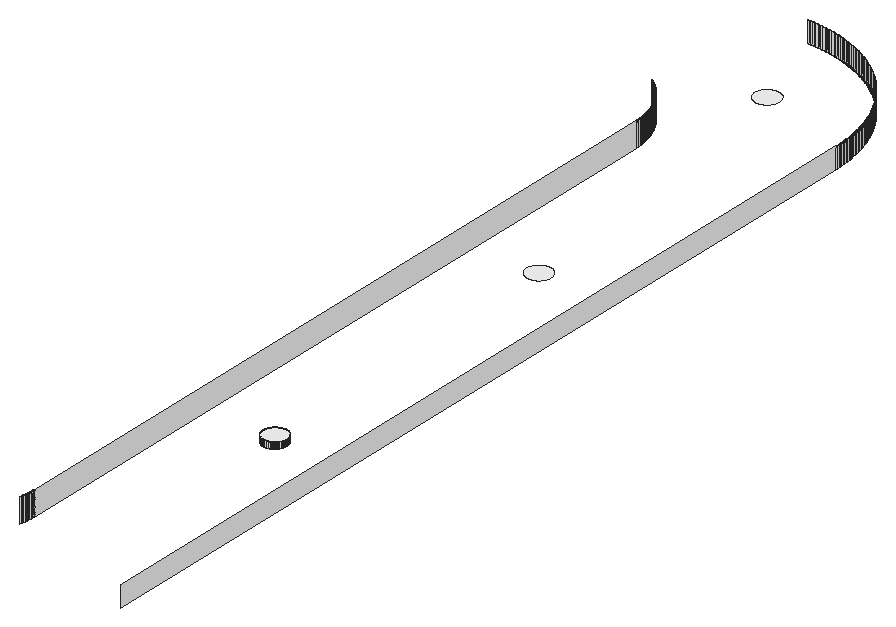
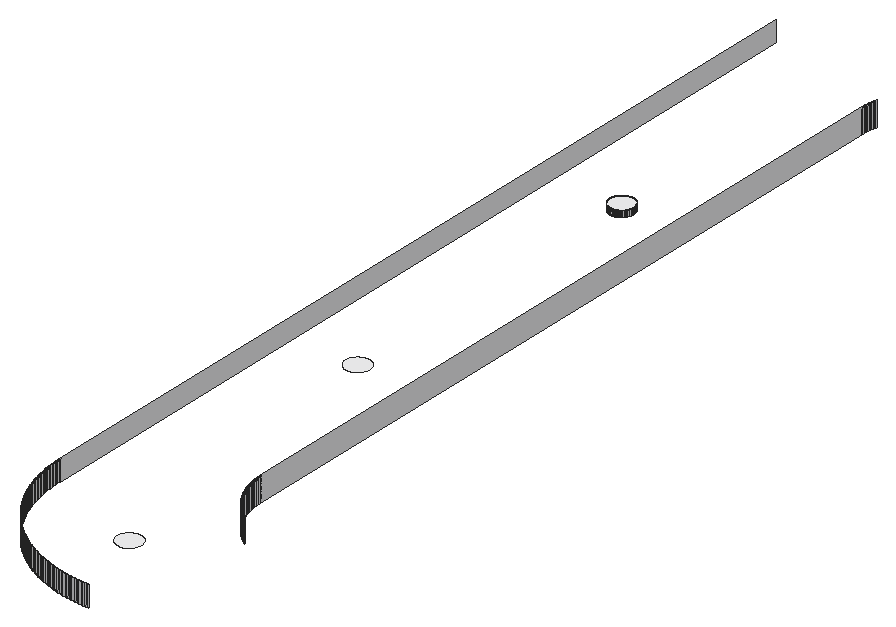
# SketchUp Ruby script. Lengths in inches.
U = 1.inch
M = Sketchup.active_model
def pt(a) = Geom::Point3d.new(a.map { |v| v * U })
def face(e, loops, mat)
  f = e.add_face(loops[0].map { |a| pt(a) })
  loops[1..].each { |l| e.add_face(l.map { |a| pt(a) }).erase! }
  f.material = f.back_material = mat if mat
  f
end
# faces: each face lists its corners as indices into pts; further lists are holes
def faces(e, pts, list, mat = nil) = list.each { |f| face(e, (f[0].is_a?(Array) ? f : [f]).map { |l| l.map { |i| pts[i] } }, mat) }
# xy, xz, yz: faces in a plane at the given z, y or x. An outline is a flat list of corners, or four numbers for a rectangle; further outlines are holes
def ring(l) = l.size == 4 ? [[l[0], l[1]], [l[2], l[1]], [l[2], l[3]], [l[0], l[3]]] : l.each_slice(2).to_a
def flat(e, list, mat, &to3) = list.each { |f| face(e, (f[0].is_a?(Array) ? f : [f]).map { |l| ring(l).map { |u, v| to3.(u, v) } }, mat) }
def xy(e, z, list, mat = nil) = flat(e, list, mat) { |x, y| [x, y, z] }
def xz(e, y, list, mat = nil) = flat(e, list, mat) { |x, z| [x, y, z] }
def yz(e, x, list, mat = nil) = flat(e, list, mat) { |y, z| [x, y, z] }
def lines(e, pts, list) = list.each { |a, b| e.add_line(pt(pts[a]), pt(pts[b])) }
# prism: a flat outline (further loops are holes) pulled along v
def prism(e, loops, v, mat = nil)
  f = face(e, loops, mat); d = Geom::Vector3d.new(v.map { |x| x * U })
  f.pushpull(f.normal.samedirection?(d) ? d.length : -d.length)
end
def box(e, o, s, mat = nil) = prism(e, [[o, [o[0] + s[0], o[1], o[2]], [o[0] + s[0], o[1] + s[1], o[2]], [o[0], o[1] + s[1], o[2]]]], [0, 0, s[2]], mat)
def at(x, y, z, deg = 0) = Geom::Transformation.translation(pt([x, y, z])) * Geom::Transformation.rotation(ORIGIN, Z_AXIS, deg.degrees)
def axes(o, x, y, z) = Geom::Transformation.new([*x, 0, *y, 0, *z, 0, *pt(o).to_a, 1])
def part(name) = M.definitions.add(name)
# library, detail: a bought-in or finely detailed component or shape, given as its bounding box
def library(name, o, s) = part(name).tap { |d| box(d.entities, o, s) }
def detail(e, o, s) = box(e.add_group.entities, o, s)
def put(e, d, t, mat = nil) = e.add_instance(d, t).tap { |i| i.material = mat if mat }
def group(e, t, mat = nil) = e.add_group.tap { |g| g.transformation = t; g.material = mat if mat }.entities
root = M.entities
M.materials.add("[Quartz Light Grey]").color = [251, 251, 252]
xy(root,112.81,[[188.98,111.35,188.85,111.36,188.73,111.37,188.6,111.39,188.48,111.42,188.24,111.5,188.13,111.55,188.02,111.61,187.91,111.68,187.81,111.75,187.71,111.83,187.62,111.91,187.53,112,187.37,112.2,187.3,112.3,187.18,112.52,187.13,112.64,187.09,112.76,187.03,113,187.01,113.125,187,113.25,187,113.375,187.02,113.625,187.04,113.75,187.1,113.99,187.2,114.23,187.26,114.34,187.32,114.44,187.39,114.55,187.47,114.65,187.65,114.83,187.74,114.91,187.84,114.98,188.06,115.12,188.28,115.22,188.52,115.3,188.65,115.32,188.77,115.34,188.9,115.35,189.15,115.35,189.27,115.34,189.4,115.31,189.52,115.29,189.76,115.21,189.87,115.15,189.98,115.1,190.09,115.03,190.19,114.96,190.29,114.88,190.38,114.8,190.47,114.71,190.63,114.51,190.7,114.41,190.76,114.3,190.82,114.1875,190.87,114.07,190.91,113.95,190.97,113.71,190.99,113.58,191,113.46,191,113.33,190.99,113.21,190.98,113.08,190.96,112.96,190.9,112.72,190.8,112.48,190.68,112.26,190.61,112.16,190.53,112.0625,190.44,111.97,190.35,111.88,190.26,111.8,190.16,111.72,190.05,111.65,189.94,111.59,189.72,111.49,189.48,111.41,189.35,111.39,189.23,111.37,189.1,111.36],[188.85,166.71,188.73,166.73,188.6,166.75,188.48,166.78,188.36,166.8125,188.24,166.86,188.13,166.91,187.91,167.03,187.81,167.1,187.71,167.18,187.53,167.36,187.45,167.45,187.37,167.55,187.3,167.66,187.24,167.76,187.18,167.875,187.13,167.99,187.09,168.11,187.03,168.35,187.01,168.48,187,168.6,187,168.73,187.01,168.86,187.02,168.98,187.04,169.1,187.07,169.23,187.1,169.35,187.15,169.46,187.2,169.58,187.32,169.8,187.39,169.9,187.47,170,187.65,170.18,187.74,170.26,187.84,170.34,187.95,170.41,188.17,170.53,188.28,170.58,188.4,170.62,188.52,170.65,188.65,170.68,188.77,170.7,188.9,170.71,189.02,170.71,189.15,170.7,189.27,170.69,189.4,170.67,189.52,170.64,189.76,170.56,189.87,170.51,190.09,170.39,190.19,170.3125,190.29,170.24,190.38,170.15,190.47,170.0625,190.55,169.97,190.63,169.87,190.7,169.76,190.82,169.54,190.87,169.42,190.91,169.31,190.94,169.19,190.97,169.0625,190.99,168.9375,191,168.8125,191,168.6875,190.98,168.4375,190.96,168.3125,190.93,168.19,190.9,168.07,190.85,167.95,190.8,167.84,190.68,167.62,190.61,167.52,190.53,167.42,190.44,167.32,190.35,167.24,190.26,167.15,190.16,167.08,190.05,167.01,189.83,166.89,189.72,166.84,189.6,166.8,189.48,166.77,189.35,166.74,189.23,166.72,189.1,166.71],[182.98,222.0625,182.85,222.07,182.73,222.08,182.6,222.1,182.48,222.13,182.24,222.21,182.13,222.26,182.02,222.32,181.91,222.39,181.81,222.46,181.71,222.54,181.62,222.62,181.53,222.71,181.45,222.8,181.37,222.9,181.3,223.01,181.18,223.23,181.13,223.35,181.09,223.47,181.03,223.71,181.01,223.83,181,223.96,181,224.08,181.01,224.21,181.02,224.33,181.04,224.46,181.1,224.7,181.15,224.82,181.2,224.93,181.26,225.05,181.32,225.15,181.39,225.26,181.47,225.35,181.56,225.45,181.65,225.54,181.74,225.62,181.84,225.69,182.06,225.83,182.28,225.93,182.52,226.01,182.65,226.03,182.77,226.05,182.9,226.06,183.02,226.0625,183.15,226.06,183.27,226.04,183.4,226.02,183.64,225.96,183.76,225.91,183.87,225.86,184.09,225.74,184.19,225.67,184.29,225.59,184.38,225.51,184.47,225.42,184.63,225.22,184.7,225.12,184.76,225.01,184.82,224.89,184.87,224.78,184.91,224.66,184.97,224.42,184.99,224.29,185,224.17,185,224.04,184.99,223.92,184.98,223.79,184.96,223.67,184.93,223.54,184.9,223.42,184.85,223.31,184.8,223.19,184.68,222.97,184.61,222.87,184.53,222.77,184.35,222.59,184.26,222.51,184.16,222.43,184.05,222.36,183.83,222.24,183.72,222.2,183.6,222.15,183.48,222.12,183.35,222.09,183.23,222.08,183.1,222.07]],"[Quartz Light Grey]")
xz(root,115.35,[[188.9,111.81,189.02,112.81],[189.02,111.81,189.15,112.81]],"[Quartz Light Grey]")
xz(root,239.99,[[177.5,111.81,177.75,115.32]],"[Quartz Light Grey]")
xz(root,240,[[177,111.81,177.25,115.32]],"[Quartz Light Grey]")
yz(root,177,[[77.6875,111.81,77.84,115.91],[77.84,111.81,78,115.91],[78,111.81,204,115.91],[204,111.81,204.16,115.91],[204.16,111.81,204.3125,115.91]],"[Quartz Light Grey]")
yz(root,187,[[113.25,111.81,113.375,112.81]],"[Quartz Light Grey]")
yz(root,191,[[113.33,111.81,113.46,112.81]],"[Quartz Light Grey]")
yz(root,200.99,[[216.5,111.81,216.75,115.32]],"[Quartz Light Grey]")
yz(root,201,[[66,111.81,216,115.32],[216,111.81,216.25,115.32]],"[Quartz Light Grey]")
p = [[176.74,75.51,111.81],[176.7,75.35,111.81],[176.7,75.35,115.91],[176.74,75.51,115.91],[176.77,75.66,111.81],[176.77,75.66,115.91],
  [176.8,75.8125,111.81],[176.8,75.8125,115.91],[176.83,75.97,111.81],[176.83,75.97,115.91],[176.85,76.12,111.81],[176.85,76.12,115.91],
  [176.875,76.28,111.81],[176.875,76.28,115.91],[176.9,76.43,111.81],[176.9,76.43,115.91],[176.92,76.59,111.81],[176.92,76.59,115.91],
  [176.93,76.75,111.81],[176.93,76.75,115.91],[176.95,76.9,111.81],[176.95,76.9,115.91],[176.96,77.06,111.81],[176.96,77.06,115.91],
  [176.97,77.22,111.81],[176.97,77.22,115.91],[176.98,77.37,111.81],[176.98,77.37,115.91],[176.99,77.53,111.81],[176.99,77.53,115.91],
  [177,77.6875,111.81],[177,77.6875,115.91],[188.48,111.42,111.81],[188.36,111.46,111.81],[188.36,111.46,112.81],[188.48,111.42,112.81],
  [188.6,111.39,111.81],[188.6,111.39,112.81],[188.73,111.37,111.81],[188.73,111.37,112.81],[188.85,111.36,111.81],[188.85,111.36,112.81],
  [188.98,111.35,111.81],[188.98,111.35,112.81],[189.1,111.36,111.81],[189.1,111.36,112.81],[189.23,111.37,111.81],[189.23,111.37,112.81],
  [189.35,111.39,111.81],[189.35,111.39,112.81],[189.48,111.41,111.81],[189.48,111.41,112.81],[189.6,111.45,111.81],[189.6,111.45,112.81],
  [189.72,111.49,111.81],[189.72,111.49,112.81],[188.24,111.5,111.81],[188.13,111.55,111.81],[188.13,111.55,112.81],[188.24,111.5,112.81],
  [189.83,111.54,111.81],[189.83,111.54,112.81],[189.94,111.59,111.81],[189.94,111.59,112.81],[188.02,111.61,111.81],[187.91,111.68,111.81],
  [187.91,111.68,112.81],[188.02,111.61,112.81],[190.05,111.65,111.81],[190.05,111.65,112.81],[187.81,111.75,111.81],[187.71,111.83,111.81],
  [187.71,111.83,112.81],[187.81,111.75,112.81],[190.16,111.72,111.81],[190.16,111.72,112.81],[190.26,111.8,111.81],[190.26,111.8,112.81],
  [187.62,111.91,111.81],[187.62,111.91,112.81],[190.35,111.88,111.81],[190.35,111.88,112.81],[187.53,112,111.81],[187.53,112,112.81],
  [190.44,111.97,111.81],[190.44,111.97,112.81],[187.45,112.1,111.81],[187.45,112.1,112.81],[190.53,112.0625,111.81],[190.53,112.0625,112.81],
  [187.37,112.2,111.81],[187.37,112.2,112.81],[190.61,112.16,111.81],[190.61,112.16,112.81],[187.3,112.3,111.81],[187.3,112.3,112.81],
  [190.68,112.26,111.81],[190.68,112.26,112.81],[187.24,112.41,111.81],[187.24,112.41,112.81],[190.74,112.37,111.81],[190.74,112.37,112.81],
  [187.18,112.52,111.81],[187.18,112.52,112.81],[190.8,112.48,111.81],[190.8,112.48,112.81],[187.13,112.64,111.81],[187.13,112.64,112.81],
  [190.85,112.6,111.81],[190.85,112.6,112.81],[187.09,112.76,111.81],[187.09,112.76,112.81],[190.9,112.72,111.81],[190.9,112.72,112.81],
  [190.93,112.84,111.81],[190.93,112.84,112.81],[187.06,112.88,111.81],[187.06,112.88,112.81],[190.96,112.96,111.81],[190.96,112.96,112.81],
  [187.03,113,111.81],[187.03,113,112.81],[187.01,113.125,111.81],[187.01,113.125,112.81],[190.98,113.08,111.81],[190.98,113.08,112.81],
  [187,113.25,111.81],[187,113.25,112.81],[190.99,113.21,111.81],[190.99,113.21,112.81],[191,113.33,111.81],[191,113.33,112.81],
  [187,113.375,111.81],[187.01,113.5,111.81],[187.01,113.5,112.81],[187,113.375,112.81],[187.02,113.625,111.81],[187.02,113.625,112.81],
  [190.99,113.58,111.81],[191,113.46,111.81],[191,113.46,112.81],[190.99,113.58,112.81],[187.04,113.75,111.81],[187.04,113.75,112.81],
  [190.97,113.71,111.81],[190.97,113.71,112.81],[190.94,113.83,111.81],[190.94,113.83,112.81],[187.07,113.87,111.81],[187.07,113.87,112.81],
  [190.91,113.95,111.81],[190.91,113.95,112.81],[187.1,113.99,111.81],[187.1,113.99,112.81],[187.15,114.11,111.81],[187.15,114.11,112.81],
  [190.87,114.07,111.81],[190.87,114.07,112.81],[187.2,114.23,111.81],[187.2,114.23,112.81],[190.82,114.1875,111.81],[190.82,114.1875,112.81],
  [187.26,114.34,111.81],[187.26,114.34,112.81],[190.76,114.3,111.81],[190.76,114.3,112.81],[187.32,114.44,111.81],[187.32,114.44,112.81],
  [190.7,114.41,111.81],[190.7,114.41,112.81],[187.39,114.55,111.81],[187.39,114.55,112.81],[190.63,114.51,111.81],[190.63,114.51,112.81],
  [187.47,114.65,111.81],[187.47,114.65,112.81],[190.55,114.61,111.81],[190.55,114.61,112.81],[187.56,114.74,111.81],[187.56,114.74,112.81],
  [190.47,114.71,111.81],[190.47,114.71,112.81],[187.65,114.83,111.81],[187.65,114.83,112.81],[190.38,114.8,111.81],[190.38,114.8,112.81],
  [187.74,114.91,111.81],[187.74,114.91,112.81],[190.29,114.88,111.81],[190.29,114.88,112.81],[187.84,114.98,111.81],[187.84,114.98,112.81],
  [190.19,114.96,111.81],[190.19,114.96,112.81],[187.95,115.05,111.81],[187.95,115.05,112.81],[189.98,115.1,111.81],[190.09,115.03,111.81],
  [190.09,115.03,112.81],[189.98,115.1,112.81],[188.06,115.12,111.81],[188.06,115.12,112.81],[188.17,115.17,111.81],[188.17,115.17,112.81],
  [189.87,115.15,111.81],[189.87,115.15,112.81],[188.28,115.22,111.81],[188.28,115.22,112.81],[188.4,115.26,111.81],[188.4,115.26,112.81],
  [189.52,115.29,111.81],[189.64,115.25,111.81],[189.64,115.25,112.81],[189.52,115.29,112.81],[189.76,115.21,111.81],[189.76,115.21,112.81],
  [188.52,115.3,111.81],[188.52,115.3,112.81],[188.65,115.32,111.81],[188.65,115.32,112.81],[188.77,115.34,111.81],[188.77,115.34,112.81],
  [188.9,115.35,111.81],[188.9,115.35,112.81],[189.15,115.35,111.81],[189.27,115.34,111.81],[189.27,115.34,112.81],[189.15,115.35,112.81],
  [189.4,115.31,111.81],[189.4,115.31,112.81],[176.99,204.47,111.81],[177,204.3125,111.81],[177,204.3125,115.91],[176.99,204.47,115.91],
  [176.98,204.63,111.81],[176.98,204.63,115.91],[176.97,204.78,111.81],[176.97,204.78,115.91],[176.96,204.94,111.81],[176.96,204.94,115.91],
  [176.95,205.1,111.81],[176.95,205.1,115.91],[176.93,205.25,111.81],[176.93,205.25,115.91],[176.92,205.41,111.81],[176.92,205.41,115.91],
  [176.9,205.57,111.81],[176.9,205.57,115.91],[176.875,205.72,111.81],[176.875,205.72,115.91],[176.85,205.88,111.81],[176.85,205.88,115.91],
  [176.83,206.03,111.81],[176.83,206.03,115.91],[176.8,206.1875,111.81],[176.8,206.1875,115.91],[176.77,206.34,111.81],[176.77,206.34,115.91],
  [176.74,206.49,111.81],[176.74,206.49,115.91],[176.7,206.65,111.81],[176.7,206.65,115.91],[176.67,206.8,111.81],[176.67,206.8,115.91],
  [176.63,206.95,111.81],[176.63,206.95,115.91],[176.59,207.11,111.81],[176.59,207.11,115.91],[176.55,207.26,111.81],[176.55,207.26,115.91],
  [176.51,207.41,111.81],[176.51,207.41,115.91],[176.46,207.56,111.81],[176.46,207.56,115.91],[176.41,207.71,111.81],[176.41,207.71,115.91],
  [176.36,207.86,111.81],[176.36,207.86,115.91],[176.3125,208.01,111.81],[176.3125,208.01,115.91],[176.26,208.15,111.81],[176.26,208.15,115.91],
  [176.2,208.3,111.81],[176.2,208.3,115.91],[176.15,208.45,111.81],[176.15,208.45,115.91],[176.09,208.59,111.81],[176.09,208.59,115.91],
  [176.03,208.74,111.81],[176.03,208.74,115.91],[175.96,208.88,111.81],[175.96,208.88,115.91],[175.9,209.02,111.81],[175.9,209.02,115.91],
  [175.83,209.17,111.81],[175.83,209.17,115.91],[175.76,209.31,111.81],[175.76,209.31,115.91],[175.69,209.45,111.81],[175.69,209.45,115.91],
  [175.62,209.59,111.81],[175.62,209.59,115.91],[175.55,209.73,111.81],[175.55,209.73,115.91],[175.47,209.86,111.81],[175.47,209.86,115.91],
  [175.39,210,111.81],[175.39,210,115.91],[175.3125,210.14,111.81],[175.3125,210.14,115.91],[175.23,210.27,111.81],[175.23,210.27,115.91],
  [175.15,210.4,111.81],[175.15,210.4,115.91],[175.0625,210.54,111.81],[175.0625,210.54,115.91],[174.98,210.67,111.81],[174.98,210.67,115.91],
  [174.89,210.8,111.81],[174.89,210.8,115.91],[174.8,210.93,111.81],[174.8,210.93,115.91],[174.71,211.05,111.81],[174.71,211.05,115.91],
  [174.62,211.18,111.81],[174.62,211.18,115.91],[174.52,211.31,111.81],[174.52,211.31,115.91],[174.42,211.43,111.81],[174.42,211.43,115.91],
  [174.33,211.55,111.81],[174.33,211.55,115.91],[174.23,211.67,111.81],[174.23,211.67,115.91],[174.125,211.79,111.81],[174.125,211.79,115.91],
  [174.02,211.91,111.81],[174.02,211.91,115.91],[173.92,212.03,111.81],[173.92,212.03,115.91],[173.8125,212.15,111.81],[173.8125,212.15,115.91],
  [173.7,212.26,111.81],[173.7,212.26,115.91],[173.6,212.375,111.81],[173.6,212.375,115.91],[173.49,212.49,111.81],[173.49,212.49,115.91],
  [173.375,212.6,111.81],[173.375,212.6,115.91],[173.26,212.7,111.81],[173.26,212.7,115.91],[173.15,212.8125,111.81],[173.15,212.8125,115.91],
  [173.03,212.92,111.81],[173.03,212.92,115.91],[172.91,213.02,111.81],[172.91,213.02,115.91],[172.79,213.125,111.81],[172.79,213.125,115.91],
  [172.67,213.23,111.81],[172.67,213.23,115.91],[172.55,213.33,111.81],[172.55,213.33,115.91],[172.43,213.42,111.81],[172.43,213.42,115.91],
  [172.31,213.52,111.81],[172.31,213.52,115.91],[172.18,213.62,111.81],[172.18,213.62,115.91],[172.05,213.71,111.81],[172.05,213.71,115.91],
  [171.93,213.8,111.81],[171.93,213.8,115.91],[171.8,213.89,111.81],[171.8,213.89,115.91],[201,216.25,111.81],[200.99,216.5,111.81],
  [200.99,216.5,115.32],[201,216.25,115.32],[200.99,216.75,111.81],[200.98,217.01,111.81],[200.98,217.01,115.32],[200.99,216.75,115.32],
  [200.97,217.26,111.81],[200.97,217.26,115.32],[200.95,217.51,111.81],[200.95,217.51,115.32],[200.9375,217.76,111.81],[200.9375,217.76,115.32],
  [200.92,218.01,111.81],[200.92,218.01,115.32],[200.89,218.26,111.81],[200.89,218.26,115.32],[200.87,218.51,111.81],[200.87,218.51,115.32],
  [200.84,218.76,111.81],[200.84,218.76,115.32],[200.8125,219.01,111.81],[200.8125,219.01,115.32],[200.78,219.26,111.81],[200.78,219.26,115.32],
  [200.74,219.51,111.81],[200.74,219.51,115.32],[200.7,219.75,111.81],[200.7,219.75,115.32],[200.66,220,111.81],[200.66,220,115.32],
  [200.62,220.25,111.81],[200.62,220.25,115.32],[200.57,220.5,111.81],[200.57,220.5,115.32],[200.53,220.74,111.81],[200.53,220.74,115.32],
  [200.48,220.99,111.81],[200.48,220.99,115.32],[200.42,221.24,111.81],[200.42,221.24,115.32],[200.37,221.48,111.81],[200.37,221.48,115.32],
  [200.31,221.72,111.81],[200.31,221.72,115.32],[200.25,221.97,111.81],[200.25,221.97,115.32],[200.18,222.21,111.81],[200.18,222.21,115.32],
  [200.12,222.45,111.81],[200.12,222.45,115.32],[200.05,222.7,111.81],[200.05,222.7,115.32],[199.98,222.9375,111.81],[199.98,222.9375,115.32],
  [199.9,223.18,111.81],[199.9,223.18,115.32],[199.83,223.42,111.81],[199.83,223.42,115.32],[199.75,223.66,111.81],[199.75,223.66,115.32],
  [199.67,223.89,111.81],[199.67,223.89,115.32],[199.58,224.13,111.81],[199.58,224.13,115.32],[199.49,224.37,111.81],[199.49,224.37,115.32],
  [199.41,224.6,111.81],[199.41,224.6,115.32],[199.31,224.83,111.81],[199.31,224.83,115.32],[199.22,225.07,111.81],[199.22,225.07,115.32],
  [199.125,225.3,111.81],[199.125,225.3,115.32],[199.03,225.53,111.81],[199.03,225.53,115.32],[198.93,225.76,111.81],[198.93,225.76,115.32],
  [198.82,225.99,111.81],[198.82,225.99,115.32],[198.72,226.22,111.81],[198.72,226.22,115.32],[198.61,226.45,111.81],[198.61,226.45,115.32],
  [198.5,226.67,111.81],[198.5,226.67,115.32],[198.38,226.9,111.81],[198.38,226.9,115.32],[198.27,227.12,111.81],[198.27,227.12,115.32],
  [198.15,227.34,111.81],[198.15,227.34,115.32],[198.03,227.5625,111.81],[198.03,227.5625,115.32],[197.91,227.78,111.81],[197.91,227.78,115.32],
  [197.78,228,111.81],[197.78,228,115.32],[197.66,228.22,111.81],[197.66,228.22,115.32],[197.53,228.43,111.81],[197.53,228.43,115.32],
  [197.4,228.65,111.81],[197.4,228.65,115.32],[197.26,228.86,111.81],[197.26,228.86,115.32],[197.13,229.07,111.81],[197.13,229.07,115.32],
  [196.99,229.28,111.81],[196.99,229.28,115.32],[196.85,229.49,111.81],[196.85,229.49,115.32],[196.71,229.7,111.81],[196.71,229.7,115.32],
  [196.5625,229.9,111.81],[196.5625,229.9,115.32],[196.42,230.11,111.81],[196.42,230.11,115.32],[196.27,230.31,111.81],[196.27,230.31,115.32],
  [196.12,230.51,111.81],[196.12,230.51,115.32],[195.96,230.71,111.81],[195.96,230.71,115.32],[195.81,230.91,111.81],[195.81,230.91,115.32],
  [195.65,231.1,111.81],[195.65,231.1,115.32],[195.49,231.3,111.81],[195.49,231.3,115.32],[195.33,231.49,111.81],[195.33,231.49,115.32],
  [195.17,231.68,111.81],[195.17,231.68,115.32],[195,231.87,111.81],[195,231.87,115.32],[194.84,232.06,111.81],[194.84,232.06,115.32],
  [194.67,232.25,111.81],[194.67,232.25,115.32],[194.5,232.43,111.81],[194.5,232.43,115.32],[194.32,232.61,111.81],[194.32,232.61,115.32],
  [194.15,232.79,111.81],[194.15,232.79,115.32],[193.97,232.97,111.81],[193.97,232.97,115.32],[193.79,233.15,111.81],[193.79,233.15,115.32],
  [193.61,233.32,111.81],[193.61,233.32,115.32],[193.43,233.5,111.81],[193.43,233.5,115.32],[193.25,233.67,111.81],[193.25,233.67,115.32],
  [193.06,233.84,111.81],[193.06,233.84,115.32],[192.87,234,111.81],[192.87,234,115.32],[192.68,234.17,111.81],[192.68,234.17,115.32],
  [192.49,234.33,111.81],[192.49,234.33,115.32],[192.3,234.49,111.81],[192.3,234.49,115.32],[192.1,234.65,111.81],[192.1,234.65,115.32],
  [191.91,234.81,111.81],[191.91,234.81,115.32],[191.71,234.96,111.81],[191.71,234.96,115.32],[191.51,235.12,111.81],[191.51,235.12,115.32],
  [191.31,235.27,111.81],[191.31,235.27,115.32],[191.11,235.42,111.81],[191.11,235.42,115.32],[190.9,235.5625,111.81],[190.9,235.5625,115.32],
  [190.7,235.71,111.81],[190.7,235.71,115.32],[190.49,235.85,111.81],[190.49,235.85,115.32],[190.28,235.99,111.81],[190.28,235.99,115.32],
  [190.07,236.13,111.81],[190.07,236.13,115.32],[189.86,236.26,111.81],[189.86,236.26,115.32],[189.65,236.4,111.81],[189.65,236.4,115.32],
  [189.43,236.53,111.81],[189.43,236.53,115.32],[189.22,236.66,111.81],[189.22,236.66,115.32],[189,236.78,111.81],[189,236.78,115.32],
  [188.78,236.91,111.81],[188.78,236.91,115.32],[188.5625,237.03,111.81],[188.5625,237.03,115.32],[188.34,237.15,111.81],[188.34,237.15,115.32],
  [188.12,237.27,111.81],[188.12,237.27,115.32],[187.9,237.38,111.81],[187.9,237.38,115.32],[187.67,237.5,111.81],[187.67,237.5,115.32],
  [187.45,237.61,111.81],[187.45,237.61,115.32],[187.22,237.72,111.81],[187.22,237.72,115.32],[186.99,237.82,111.81],[186.99,237.82,115.32],
  [186.76,237.93,111.81],[186.76,237.93,115.32],[186.53,238.03,111.81],[186.53,238.03,115.32],[186.3,238.125,111.81],[186.3,238.125,115.32],
  [186.07,238.22,111.81],[186.07,238.22,115.32],[185.83,238.31,111.81],[185.83,238.31,115.32],[185.6,238.41,111.81],[185.6,238.41,115.32],
  [185.37,238.49,111.81],[185.37,238.49,115.32],[185.13,238.58,111.81],[185.13,238.58,115.32],[184.89,238.67,111.81],[184.89,238.67,115.32],
  [184.66,238.75,111.81],[184.42,238.83,111.81],[184.42,238.83,115.32],[184.66,238.75,115.32],[184.18,238.9,111.81],[184.18,238.9,115.32],
  [183.9375,238.98,111.81],[183.9375,238.98,115.32],[183.7,239.05,111.81],[183.45,239.12,111.81],[183.45,239.12,115.32],[183.7,239.05,115.32],
  [183.21,239.18,111.81],[183.21,239.18,115.32],[182.97,239.25,111.81],[182.72,239.31,111.81],[182.72,239.31,115.32],[182.97,239.25,115.32],
  [182.48,239.37,111.81],[182.48,239.37,115.32],[182.24,239.42,111.81],[181.99,239.48,111.81],[181.99,239.48,115.32],[182.24,239.42,115.32],
  [181.74,239.53,111.81],[181.5,239.57,111.81],[181.5,239.57,115.32],[181.74,239.53,115.32],[181.25,239.62,111.81],[181,239.66,111.81],
  [181,239.66,115.32],[181.25,239.62,115.32],[180.51,239.74,111.81],[180.26,239.78,111.81],[180.26,239.78,115.32],[180.51,239.74,115.32],
  [180.75,239.7,111.81],[180.75,239.7,115.32],[179.76,239.84,111.81],[179.51,239.87,111.81],[179.51,239.87,115.32],[179.76,239.84,115.32],
  [180.01,239.8125,111.81],[180.01,239.8125,115.32],[178.76,239.9375,111.81],[178.51,239.95,111.81],[178.51,239.95,115.32],[178.76,239.9375,115.32],
  [179.01,239.92,111.81],[179.01,239.92,115.32],[179.26,239.89,111.81],[179.26,239.89,115.32],[177.5,239.99,111.81],[177.25,240,111.81],
  [177.25,240,115.32],[177.5,239.99,115.32],[178.01,239.98,111.81],[177.75,239.99,111.81],[177.75,239.99,115.32],[178.01,239.98,115.32],
  [178.26,239.97,111.81],[178.26,239.97,115.32]]
faces(root,p,[[0,1,2,3],[4,0,3,5],[6,4,5,7],[8,6,7,9],[10,8,9,11],[12,10,11,13],[14,12,13,15],[16,14,15,17],
  [18,16,17,19],[20,18,19,21],[22,20,21,23],[24,22,23,25],[26,24,25,27],[28,26,27,29],[30,28,29,31],[32,33,34,35],
  [36,32,35,37],[38,36,37,39],[40,38,39,41],[42,40,41,43],[44,42,43,45],[46,44,45,47],[48,46,47,49],[50,48,49,51],
  [52,50,51,53],[54,52,53,55],[56,57,58,59],[33,56,59,34],[60,54,55,61],[62,60,61,63],[64,65,66,67],[57,64,67,58],
  [68,62,63,69],[70,71,72,73],[65,70,73,66],[74,68,69,75],[76,74,75,77],[71,78,79,72],[80,76,77,81],[78,82,83,79],
  [84,80,81,85],[82,86,87,83],[88,84,85,89],[86,90,91,87],[92,88,89,93],[90,94,95,91],[96,92,93,97],[94,98,99,95],
  [100,96,97,101],[98,102,103,99],[104,100,101,105],[102,106,107,103],[108,104,105,109],[106,110,111,107],[112,108,109,113],[114,112,113,115],
  [110,116,117,111],[118,114,115,119],[116,120,121,117],[120,122,123,121],[124,118,119,125],[122,126,127,123],[128,124,125,129],[130,128,129,131],
  [132,133,134,135],[133,136,137,134],[138,139,140,141],[136,142,143,137],[144,138,141,145],[146,144,145,147],[142,148,149,143],[150,146,147,151],
  [148,152,153,149],[152,154,155,153],[156,150,151,157],[154,158,159,155],[160,156,157,161],[158,162,163,159],[164,160,161,165],[162,166,167,163],
  [168,164,165,169],[166,170,171,167],[172,168,169,173],[170,174,175,171],[176,172,173,177],[174,178,179,175],[180,176,177,181],[178,182,183,179],
  [184,180,181,185],[182,186,187,183],[188,184,185,189],[186,190,191,187],[192,188,189,193],[190,194,195,191],[196,197,198,199],[197,192,193,198],
  [194,200,201,195],[200,202,203,201],[204,196,199,205],[202,206,207,203],[206,208,209,207],[210,211,212,213],[211,214,215,212],[214,204,205,215],
  [208,216,217,209],[216,218,219,217],[218,220,221,219],[220,222,223,221],[224,225,226,227],[225,228,229,226],[228,210,213,229],[230,231,232,233],
  [234,230,233,235],[236,234,235,237],[238,236,237,239],[240,238,239,241],[242,240,241,243],[244,242,243,245],[246,244,245,247],[248,246,247,249],
  [250,248,249,251],[252,250,251,253],[254,252,253,255],[256,254,255,257],[258,256,257,259],[260,258,259,261],[262,260,261,263],[264,262,263,265],
  [266,264,265,267],[268,266,267,269],[270,268,269,271],[272,270,271,273],[274,272,273,275],[276,274,275,277],[278,276,277,279],[280,278,279,281],
  [282,280,281,283],[284,282,283,285],[286,284,285,287],[288,286,287,289],[290,288,289,291],[292,290,291,293],[294,292,293,295],[296,294,295,297],
  [298,296,297,299],[300,298,299,301],[302,300,301,303],[304,302,303,305],[306,304,305,307],[308,306,307,309],[310,308,309,311],[312,310,311,313],
  [314,312,313,315],[316,314,315,317],[318,316,317,319],[320,318,319,321],[322,320,321,323],[324,322,323,325],[326,324,325,327],[328,326,327,329],
  [330,328,329,331],[332,330,331,333],[334,332,333,335],[336,334,335,337],[338,336,337,339],[340,338,339,341],[342,340,341,343],[344,342,343,345],
  [346,344,345,347],[348,346,347,349],[350,348,349,351],[352,350,351,353],[354,352,353,355],[356,354,355,357],[358,356,357,359],[360,358,359,361],
  [362,360,361,363],[364,362,363,365],[366,364,365,367],[368,366,367,369],[370,368,369,371],[372,370,371,373],[374,372,373,375],[376,377,378,379],
  [380,381,382,383],[381,384,385,382],[384,386,387,385],[386,388,389,387],[388,390,391,389],[390,392,393,391],[392,394,395,393],[394,396,397,395],
  [396,398,399,397],[398,400,401,399],[400,402,403,401],[402,404,405,403],[404,406,407,405],[406,408,409,407],[408,410,411,409],[410,412,413,411],
  [412,414,415,413],[414,416,417,415],[416,418,419,417],[418,420,421,419],[420,422,423,421],[422,424,425,423],[424,426,427,425],[426,428,429,427],
  [428,430,431,429],[430,432,433,431],[432,434,435,433],[434,436,437,435],[436,438,439,437],[438,440,441,439],[440,442,443,441],[442,444,445,443],
  [444,446,447,445],[446,448,449,447],[448,450,451,449],[450,452,453,451],[452,454,455,453],[454,456,457,455],[456,458,459,457],[458,460,461,459],
  [460,462,463,461],[462,464,465,463],[464,466,467,465],[466,468,469,467],[468,470,471,469],[470,472,473,471],[472,474,475,473],[474,476,477,475],
  [476,478,479,477],[478,480,481,479],[480,482,483,481],[482,484,485,483],[484,486,487,485],[486,488,489,487],[488,490,491,489],[490,492,493,491],
  [492,494,495,493],[494,496,497,495],[496,498,499,497],[498,500,501,499],[500,502,503,501],[502,504,505,503],[504,506,507,505],[506,508,509,507],
  [508,510,511,509],[510,512,513,511],[512,514,515,513],[514,516,517,515],[516,518,519,517],[518,520,521,519],[520,522,523,521],[522,524,525,523],
  [524,526,527,525],[526,528,529,527],[528,530,531,529],[530,532,533,531],[532,534,535,533],[534,536,537,535],[536,538,539,537],[538,540,541,539],
  [540,542,543,541],[542,544,545,543],[544,546,547,545],[546,548,549,547],[548,550,551,549],[550,552,553,551],[552,554,555,553],[554,556,557,555],
  [556,558,559,557],[558,560,561,559],[560,562,563,561],[562,564,565,563],[564,566,567,565],[566,568,569,567],[568,570,571,569],[570,572,573,571],
  [572,574,575,573],[574,576,577,575],[576,578,579,577],[578,580,581,579],[580,582,583,581],[582,584,585,583],[584,586,587,585],[586,588,589,587],
  [588,590,591,589],[590,592,593,591],[592,594,595,593],[594,596,597,595],[596,598,599,597],[598,600,601,599],[600,602,603,601],[602,604,605,603],
  [604,606,607,605],[606,608,609,607],[608,610,611,609],[612,613,614,615],[610,612,615,611],[613,616,617,614],[616,618,619,617],[620,621,622,623],
  [618,620,623,619],[621,624,625,622],[626,627,628,629],[624,626,629,625],[627,630,631,628],[632,633,634,635],[630,632,635,631],[636,637,638,639],
  [633,636,639,634],[640,641,642,643],[637,640,643,638],[644,645,646,647],[648,644,647,649],[641,648,649,642],[650,651,652,653],[654,650,653,655],
  [645,654,655,646],[656,657,658,659],[660,656,659,661],[662,660,661,663],[651,662,663,652],[664,665,666,667],[668,669,670,671],[672,668,671,673],
  [657,672,673,658]],"[Quartz Light Grey]")
